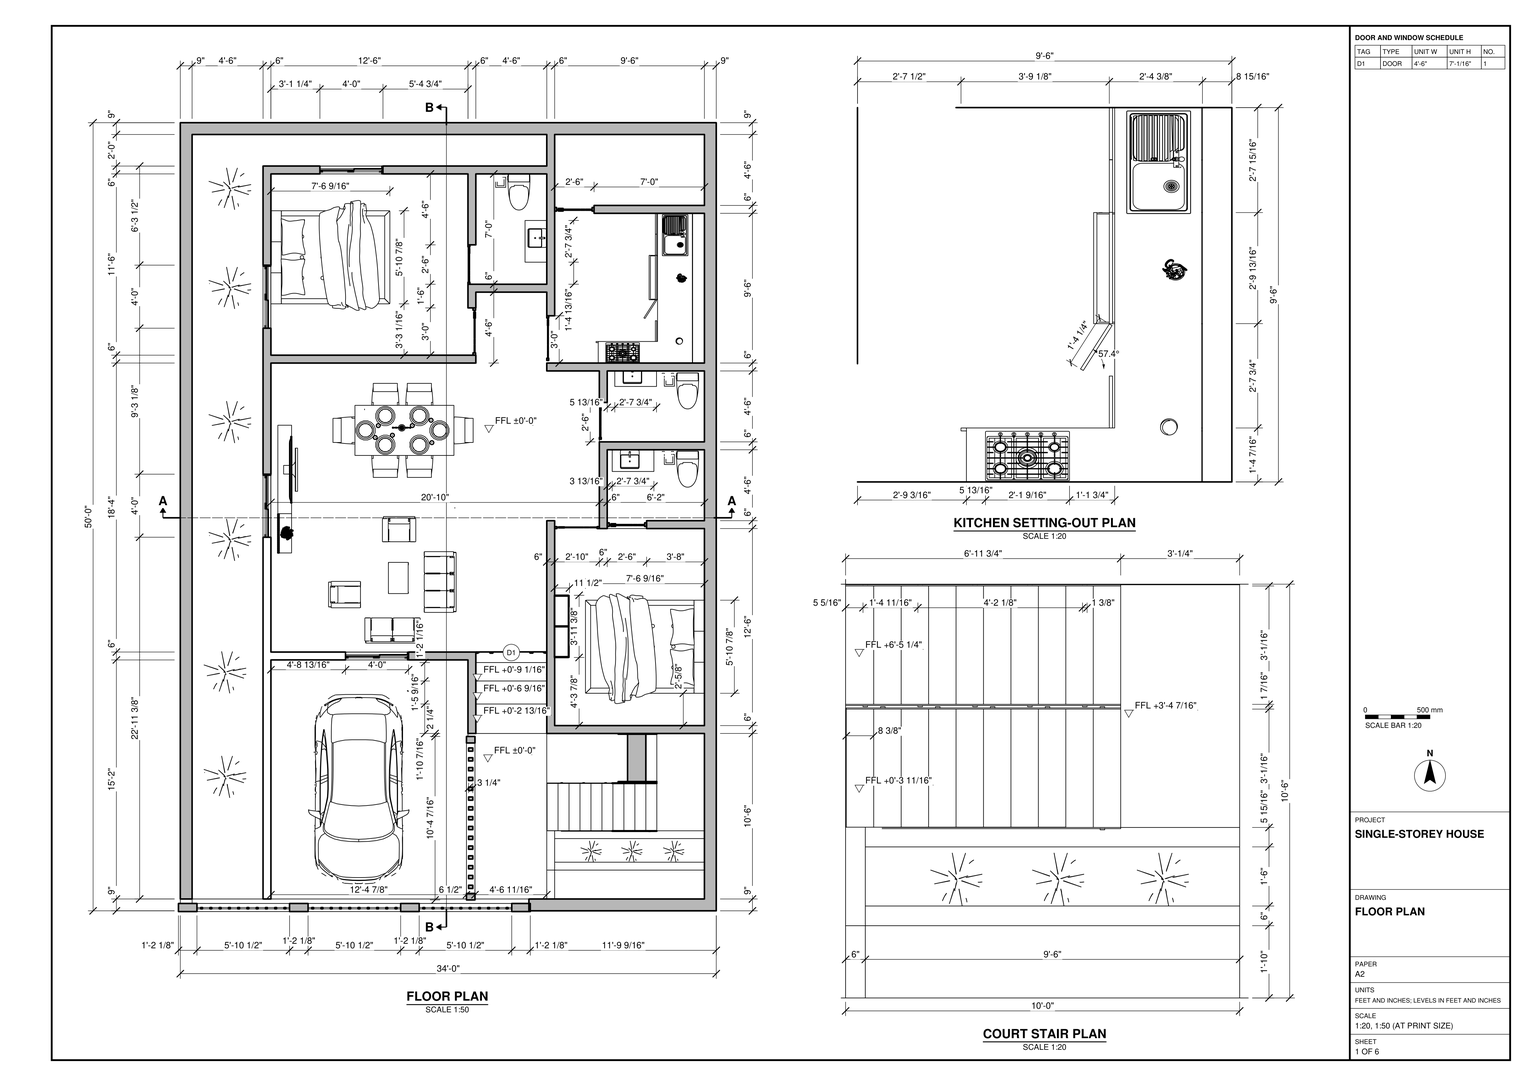
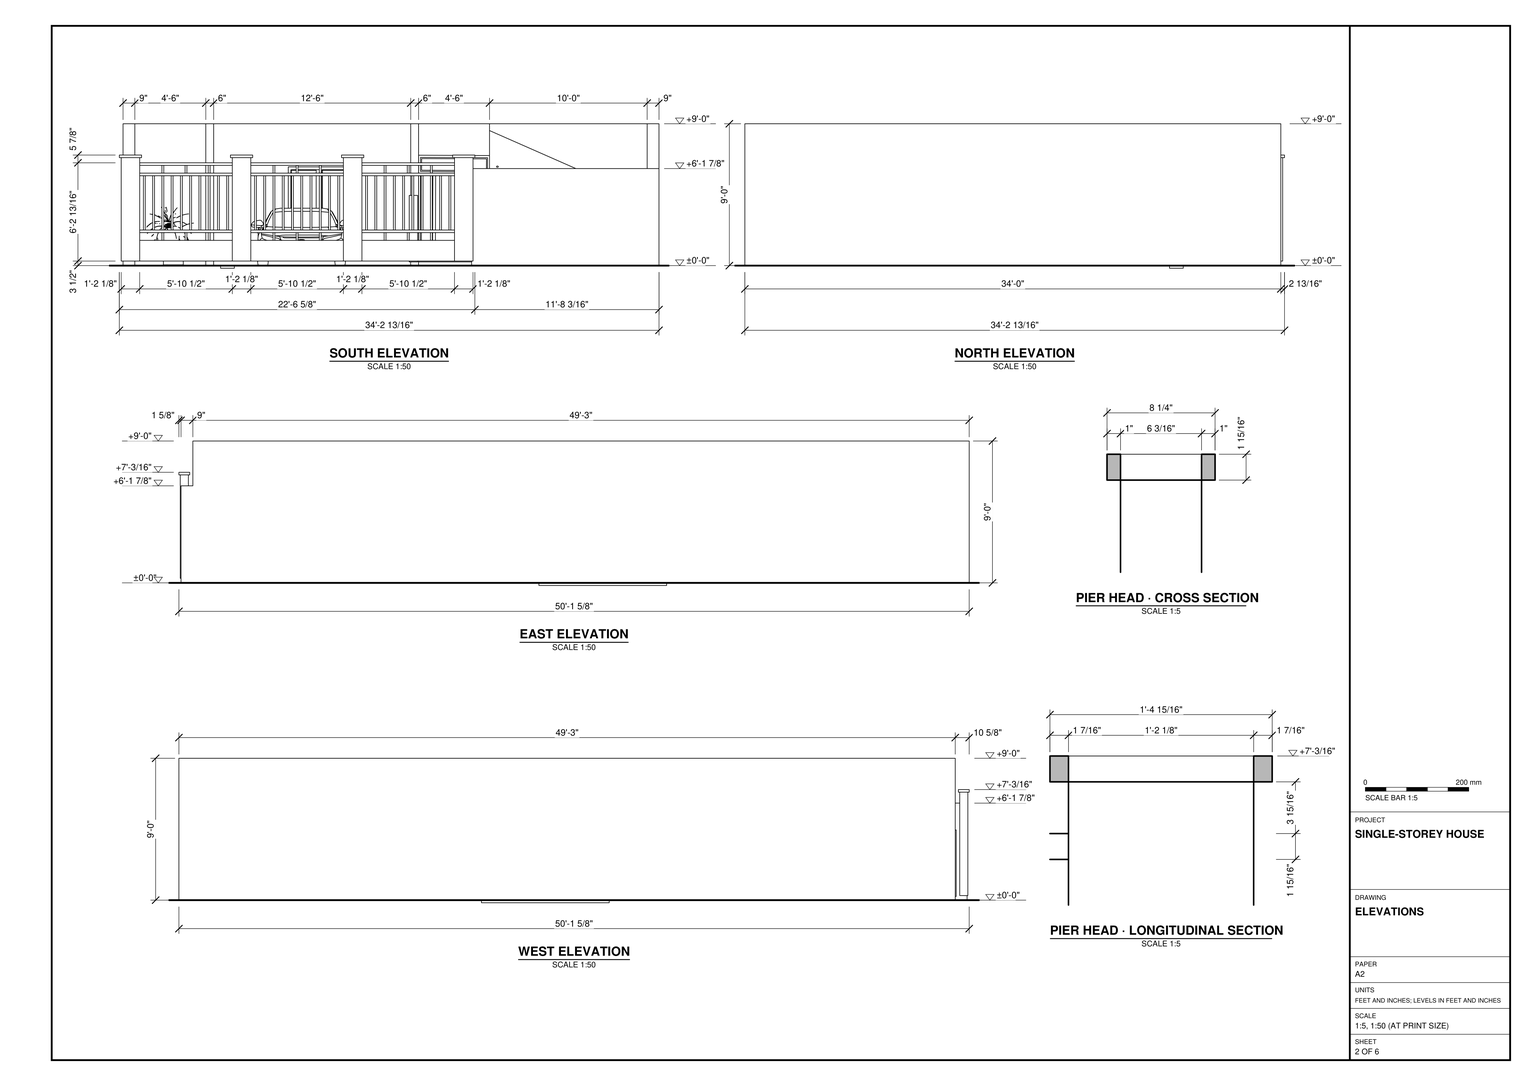
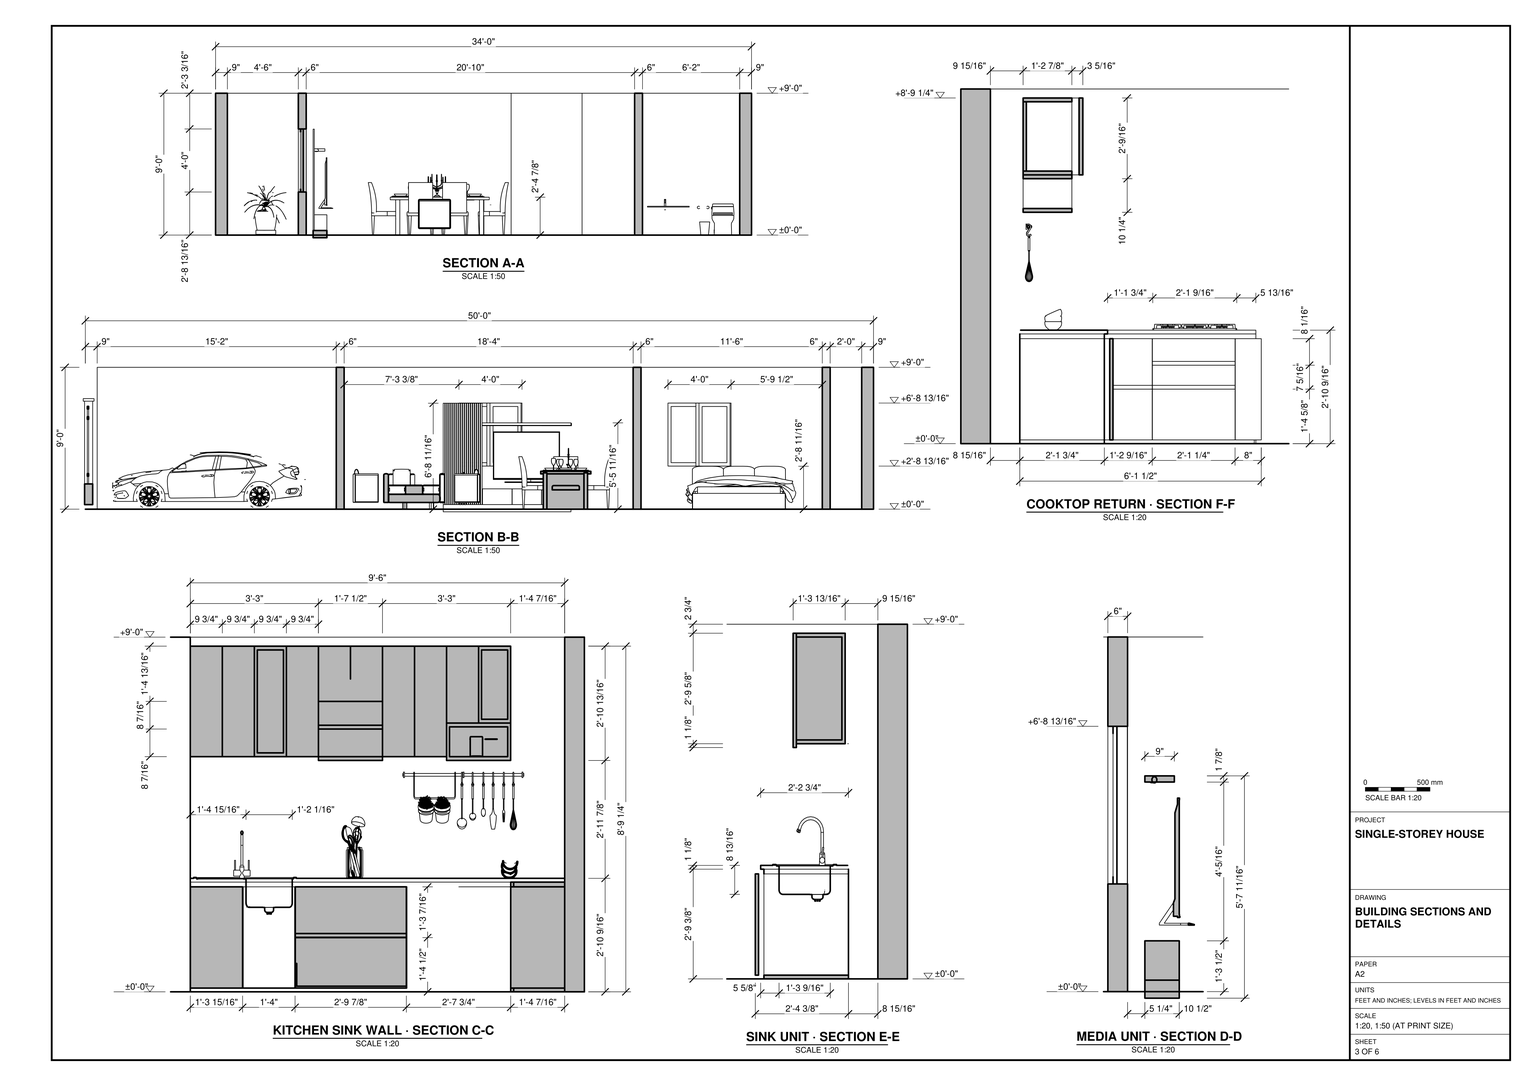
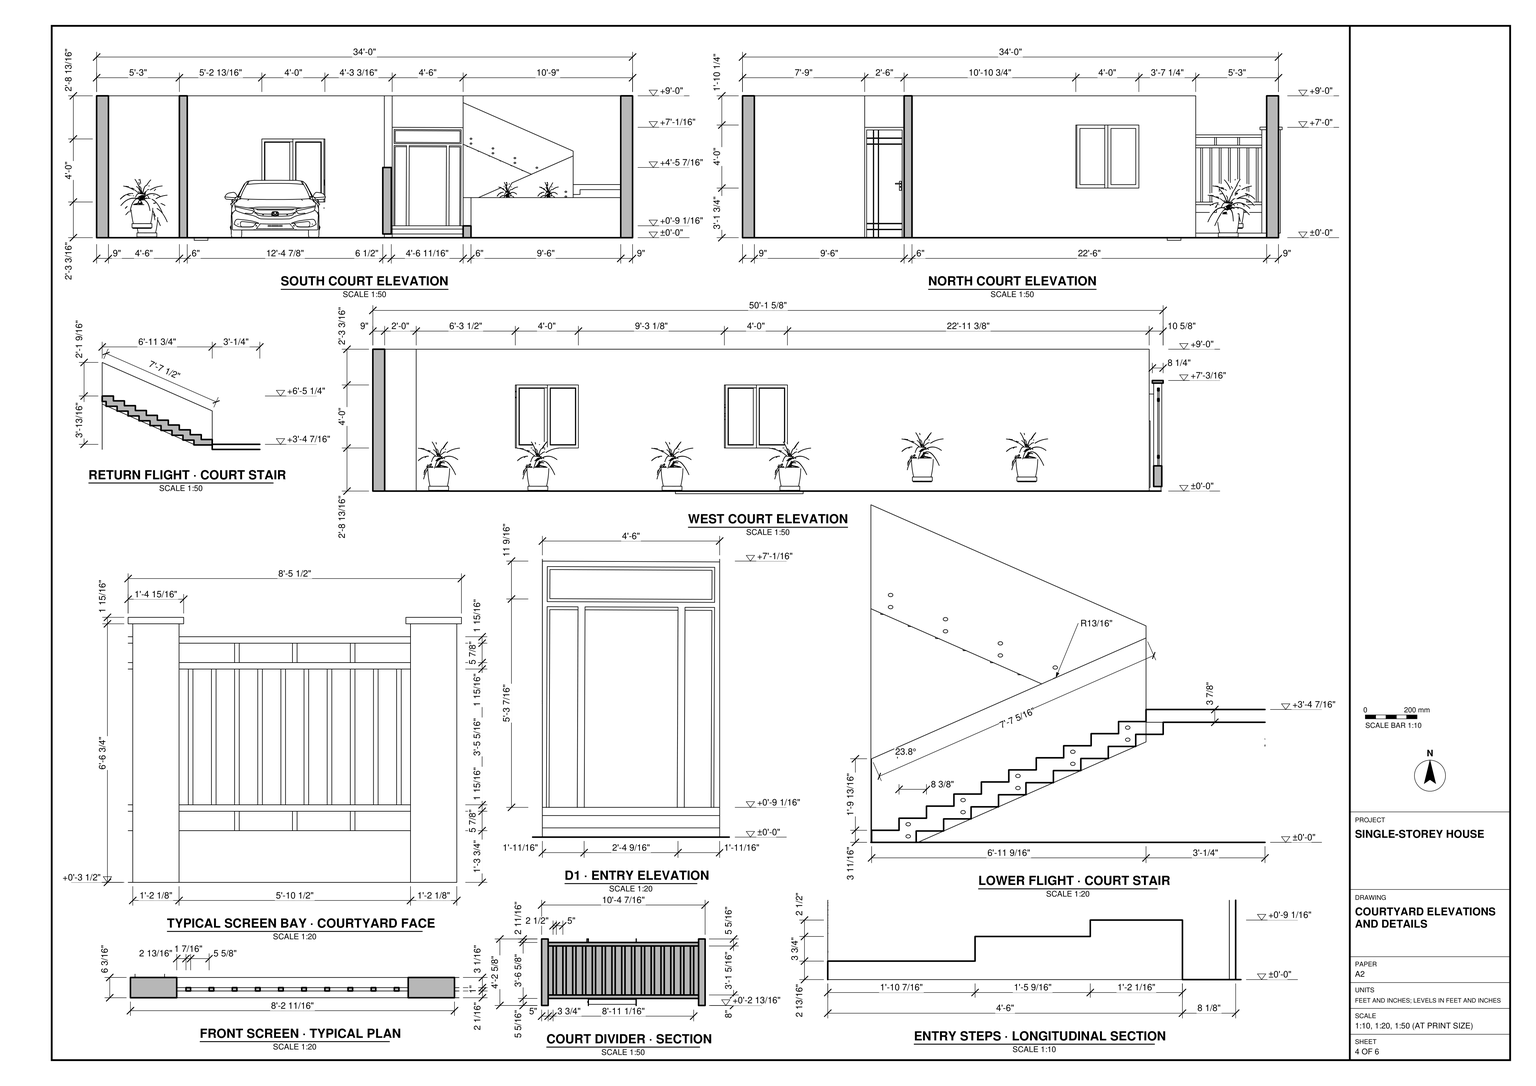
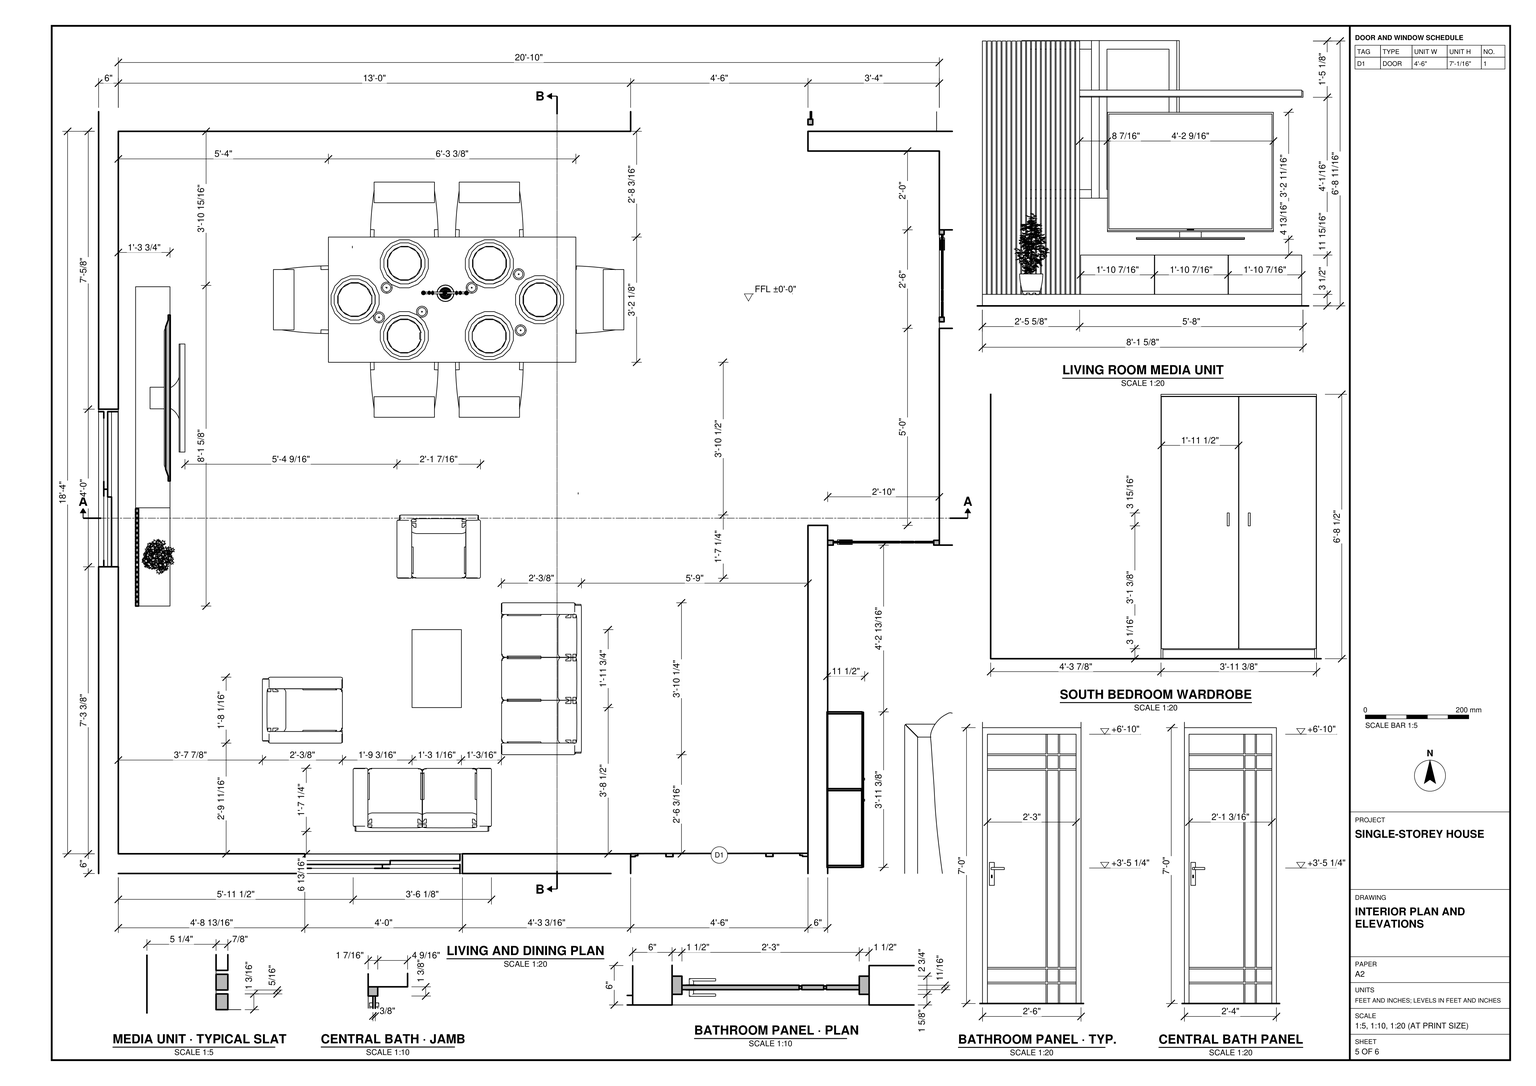
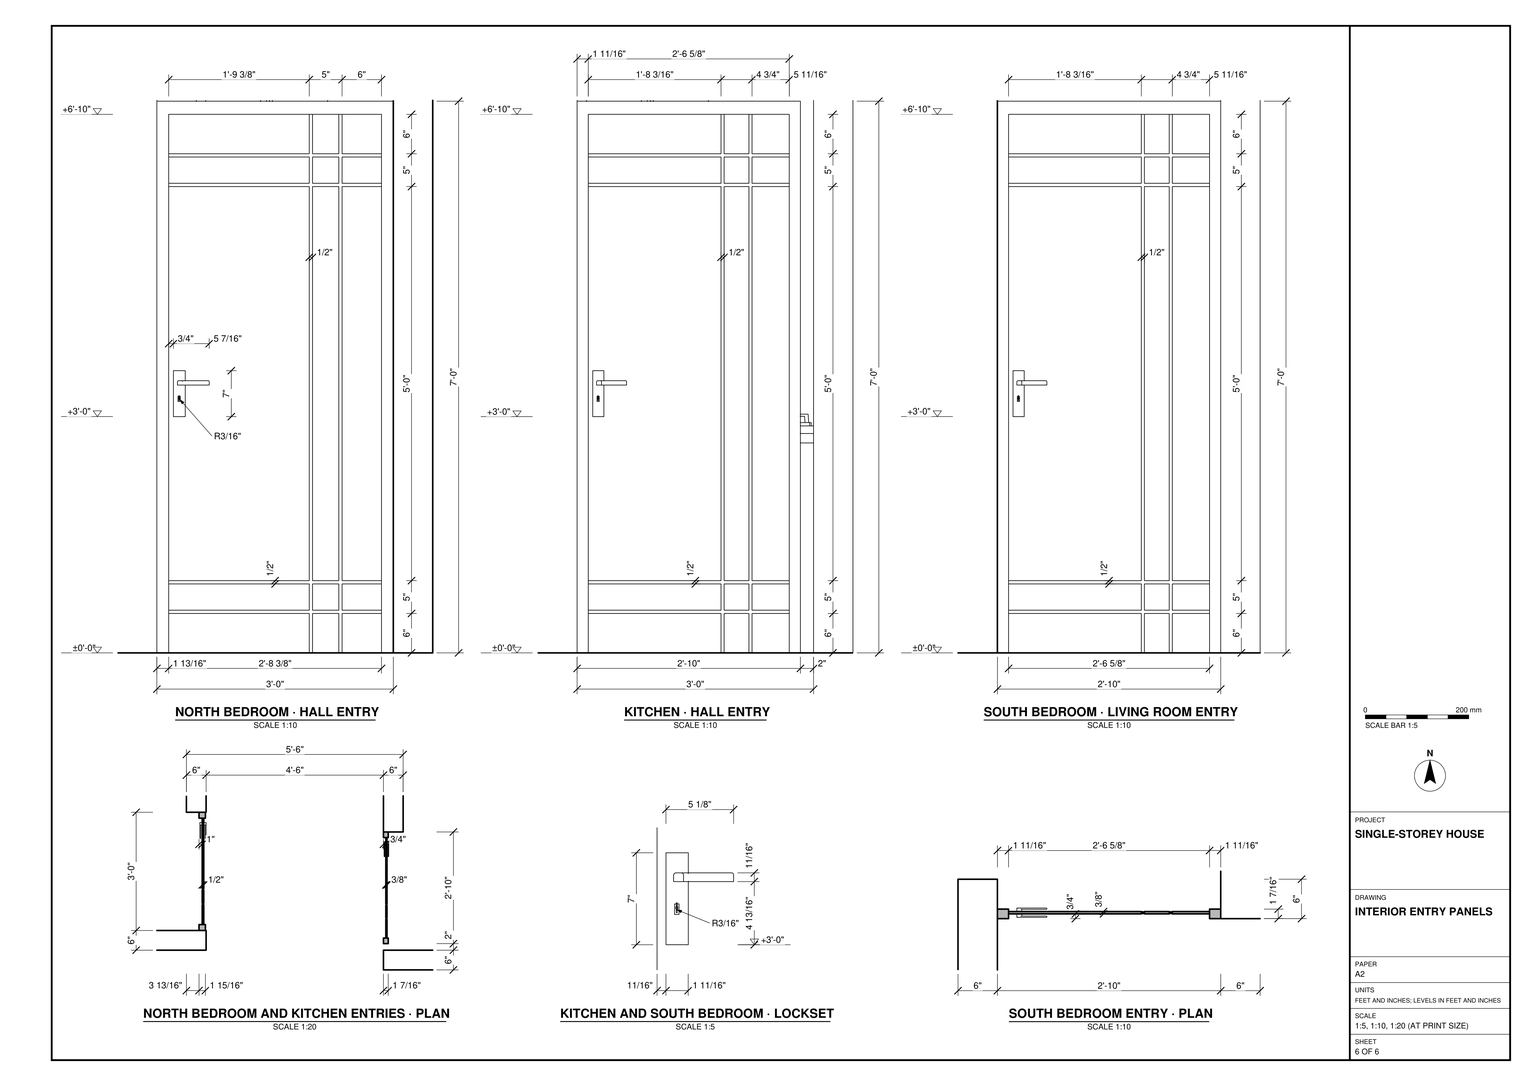
Build the house in SketchUp from task_files/diagram_01.pdf. Work in feet and inches. The complete model, including the front boundary, is 34'-2 13/16" wide, 50'-1 5/8" deep and 9'-2" high. Use ±0'-0" as the ground-floor level; the entrance steps and court stair are local changes in level, not additional storeys.

Set out the floor slabs and walls from the plan, using 9" perimeter walls and 6" partitions where dimensioned. Place the living and dining space between the two bedrooms, with the kitchen to the northeast and the sanitary rooms in their drawn positions. Fit the door and window units into the wall openings. Follow the sections for wall heads, sills and slab edges, and keep the courts open. Include the front parking bay, the planted side passage, the stepped entrance and the separate stair in the southeast court. Match the railed bays, capped piers and solid wall in the south elevation.

Model the kitchen base and wall cabinets, sink counter and cooktop return from the setting-out plan and sections. Include the beds, dining table and chairs, living-room seating, low table, media unit and sanitary fixtures at the sizes and positions shown. Decor and loose items may be any suitable library components.

Keep shell elements and individual furniture and joinery pieces in separate groups or components, and use components for repeated parts. Save one SketchUp model as output_files/single_storey_house_with_a_stair_court.skp.

# SketchUp Ruby script. Lengths in inches.
U = 1.inch
M = Sketchup.active_model
def pt(a) = Geom::Point3d.new(a.map { |v| v * U })
def face(e, loops, mat)
  f = e.add_face(loops[0].map { |a| pt(a) })
  loops[1..].each { |l| e.add_face(l.map { |a| pt(a) }).erase! }
  f.material = f.back_material = mat if mat
  f
end
# faces: each face lists its corners as indices into pts; further lists are holes
def faces(e, pts, list, mat = nil) = list.each { |f| face(e, (f[0].is_a?(Array) ? f : [f]).map { |l| l.map { |i| pts[i] } }, mat) }
# xy, xz, yz: faces in a plane at the given z, y or x. An outline is a flat list of corners, or four numbers for a rectangle; further outlines are holes
def ring(l) = l.size == 4 ? [[l[0], l[1]], [l[2], l[1]], [l[2], l[3]], [l[0], l[3]]] : l.each_slice(2).to_a
def flat(e, list, mat, &to3) = list.each { |f| face(e, (f[0].is_a?(Array) ? f : [f]).map { |l| ring(l).map { |u, v| to3.(u, v) } }, mat) }
def xy(e, z, list, mat = nil) = flat(e, list, mat) { |x, y| [x, y, z] }
def xz(e, y, list, mat = nil) = flat(e, list, mat) { |x, z| [x, y, z] }
def yz(e, x, list, mat = nil) = flat(e, list, mat) { |y, z| [x, y, z] }
def lines(e, pts, list) = list.each { |a, b| e.add_line(pt(pts[a]), pt(pts[b])) }
# prism: a flat outline (further loops are holes) pulled along v
def prism(e, loops, v, mat = nil)
  f = face(e, loops, mat); d = Geom::Vector3d.new(v.map { |x| x * U })
  f.pushpull(f.normal.samedirection?(d) ? d.length : -d.length)
end
def box(e, o, s, mat = nil) = prism(e, [[o, [o[0] + s[0], o[1], o[2]], [o[0] + s[0], o[1] + s[1], o[2]], [o[0], o[1] + s[1], o[2]]]], [0, 0, s[2]], mat)
def at(x, y, z, deg = 0) = Geom::Transformation.translation(pt([x, y, z])) * Geom::Transformation.rotation(ORIGIN, Z_AXIS, deg.degrees)
def axes(o, x, y, z) = Geom::Transformation.new([*x, 0, *y, 0, *z, 0, *pt(o).to_a, 1])
def part(name) = M.definitions.add(name)
# library, detail: a bought-in or finely detailed component or shape, given as its bounding box
def library(name, o, s) = part(name).tap { |d| box(d.entities, o, s) }
def detail(e, o, s) = box(e.add_group.entities, o, s)
def put(e, d, t, mat = nil) = e.add_instance(d, t).tap { |i| i.material = mat if mat }
def group(e, t, mat = nil) = e.add_group.tap { |g| g.transformation = t; g.material = mat if mat }.entities
root = M.entities
M.materials.add("3-Examples-of-Design-of-Three-Wooden-Entrance-Door-with-Side").color = [165, 127, 91]
M.materials.add("[Cladding Siding White]").color = [207, 207, 207]
M.materials.add("[Grass Dark Green]").color = [106, 157, 55]
M.materials.add("[Groundcover Rock Crushed Multi]").color = [143, 133, 129]
M.materials.add("[Marble Carrara Floor Tile]").color = [204, 208, 219]
M.materials.add("[Metal_Aluminum_Anodized]").color = [200, 209, 218]
M.materials.add("[Pavers Flagstone Gray]").color = [162, 162, 162]
M.materials.add("[Pavers with Grass Herringbone]").color = [197, 201, 190]
M.materials.add("[Translucent Glass Blue]").color = [100, 149, 237]
M.materials["[Translucent Glass Blue]"].alpha = 0.5
M.materials.add("[Translucent Glass Gray]").color = [128, 128, 128]
M.materials["[Translucent Glass Gray]"].alpha = 0.5
M.materials.add("[Vegetation Bark Ponderosa]").color = [158, 116, 100]
M.materials.add("[Wood Fence with Lattice]").color = [170, 106, 61]
c1 = part("Agrupar\#1")
detail(c1.entities,[0,0,0],[43.31,13.99,7.25])
c2 = library("Agrupar\#2",[0,0,0],[66.49,2.6,38.28])
c3 = part("Samsung 75")
p = [[0,0,0],[1,0,0],[1,1,0]]
lines(c3.entities,p,[[0,1],[1,2],[2,0]])
put(c3.entities,c1,at(200.625,110.82,-2.44),"[Metal_Aluminum_Anodized]")
put(c3.entities,c2,at(189.03,116.54,0))
c4 = library("Vtufgjkbc",[-37.34,-38.3,0],[76.68,71.13,141.17])
c5 = part("Enscape.LinearLight")
xz(c5.entities,-44.64,[[0,-1,0,0,-0.38,-0.92],[0,-1,0.38,-0.92,0,0],[-0.38,-0.92,0,0,-0.71,-0.71],[0.38,-0.92,0.71,-0.71,0,0],[-0.71,-0.71,0,0,-0.92,-0.38],
  [0.71,-0.71,0.92,-0.38,0,0],[-0.92,-0.38,0,0,-1,0],[0.92,-0.38,1,0,0,0],[-1,0,0,0,-0.92,0.38],[0,0,-0.71,0.71,-0.92,0.38],
  [0,0,-0.38,0.92,-0.71,0.71],[0,0,0,1,-0.38,0.92],[0,0,0.38,0.92,0,1],[0,0,0.71,0.71,0.38,0.92],[0,0,0.92,0.38,0.71,0.71],
  [0,0,1,0,0.92,0.38]])
xz(c5.entities,44.64,[[0,-1,-0.38,-0.92,0,0],[0,-1,0,0,0.38,-0.92],[-0.38,-0.92,-0.71,-0.71,0,0],[0.38,-0.92,0,0,0.71,-0.71],[-0.71,-0.71,-0.92,-0.38,0,0],
  [0.71,-0.71,0,0,0.92,-0.38],[-0.92,-0.38,-1,0,0,0],[0.92,-0.38,0,0,1,0],[-1,0,-0.92,0.38,0,0],[0,0,-0.92,0.38,-0.71,0.71],
  [0,0,-0.71,0.71,-0.38,0.92],[0,0,-0.38,0.92,0,1],[0,0,0,1,0.38,0.92],[0,0,0.38,0.92,0.71,0.71],[0,0,0.71,0.71,0.92,0.38],
  [0,0,0.92,0.38,1,0]])
p = [[-0.38,-44.64,-0.92],[-0.38,44.64,-0.92],[0,44.64,-1],[0,-44.64,-1],[0.38,44.64,-0.92],[0.38,-44.64,-0.92],
  [-0.71,-44.64,-0.71],[-0.71,44.64,-0.71],[0.71,44.64,-0.71],[0.71,-44.64,-0.71],[-0.92,-44.64,-0.38],[-0.92,44.64,-0.38],
  [0.92,44.64,-0.38],[0.92,-44.64,-0.38],[-1,-44.64,0],[-1,44.64,0],[1,44.64,0],[1,-44.64,0],
  [-0.92,-44.64,0.38],[-0.92,44.64,0.38],[0.92,44.64,0.38],[0.92,-44.64,0.38],[-0.71,-44.64,0.71],[-0.71,44.64,0.71],
  [0.71,44.64,0.71],[0.71,-44.64,0.71],[-0.38,-44.64,0.92],[-0.38,44.64,0.92],[0.38,44.64,0.92],[0.38,-44.64,0.92],
  [0,-44.64,1],[0,44.64,1]]
faces(c5.entities,p,[[0,1,2],[0,2,3],[3,2,4],[3,4,5],[6,7,1],[6,1,0],[5,4,8],[5,8,9],
  [10,11,7],[10,7,6],[9,8,12],[9,12,13],[14,15,11],[14,11,10],[13,12,16],[13,16,17],
  [18,19,15],[18,15,14],[17,16,20],[17,20,21],[22,23,19],[22,19,18],[21,20,24],[21,24,25],
  [26,27,23],[26,23,22],[25,24,28],[25,28,29],[30,31,27],[30,27,26],[29,28,31],[29,31,30]])
c6 = part("Group\#8")
box(c6.entities,[0,0,0],[1.57,1.18,81.22])
c7 = part("tv unit")
put(c7.entities,c3,at(-134.98,-45.95,38.54))
put(c7.entities,c4,axes([23.51,76.07,18.38],[0.185,0,0],[0,0.185,0],[0,0,0.185]))
put(c7.entities,c5,axes([87.75,81.2,82.67],[-0.0192,0.99911,-0.03748],[-0.99982,-0.01919,0.00072],[0,0.03749,0.9993]))
g1 = group(c7.entities,at(3.9375,84.65,12.68))
box(g1,[0,-13.78,0],[127.95,13.78,5.79])
g2 = group(c7.entities,at(43.31,84.65,18.46))
prism(g2,[[[0,0,0],[88.58,0,0],[88.58,-13.78,0],[59.21,-13.78,0],[59.21,-12.99,0],[59.06,-12.99,0],[59.06,-13.78,0],[29.69,-13.78,0],[29.69,-12.99,0],[29.53,-12.99,0],[29.53,-13.78,0],[0,-13.78,0]]],[0,0,12.6])
g3 = group(c7.entities,at(3.9375,84.65,18.46))
put(g3,c6,at(0,-1.18,0))
g4 = group(g3,at(1.97,-1.18,0))
box(g4,[0,0,0],[1.57,1.18,81.22])
put(g3,c6,at(3.9375,-1.18,0))
put(g3,c6,at(5.91,-1.18,0))
g5 = group(g3,at(7.875,-1.18,0))
box(g5,[0,0,0],[1.57,1.18,81.22])
put(g3,c6,at(9.84,-1.18,0))
put(g3,c6,at(11.8125,-1.18,0))
put(g3,c6,at(13.78,-1.18,0))
put(g3,c6,at(15.75,-1.18,0))
put(g3,c6,at(17.72,-1.18,0))
put(g3,c6,at(19.69,-1.18,0))
put(g3,c6,at(21.65,-1.18,0))
put(g3,c6,at(23.62,-1.18,0))
g6 = group(g3,at(25.59,-1.18,0))
box(g6,[0,0,0],[1.57,1.18,81.22])
put(g3,c6,at(27.56,-1.18,0))
put(g3,c6,at(29.53,-1.18,0))
put(g3,c6,at(31.5,-1.18,0))
put(g3,c6,at(33.46,-1.18,0))
put(g3,c6,at(35.43,-1.18,0))
put(g3,c6,at(37.4,-1.18,0))
g7 = group(c7.entities,at(42.91,84.65,81.97))
box(g7,[0,-11.8125,0],[88.98,11.8125,1.97])
c8 = library("Шкаф+для+одежды+1",[-0.2,0,0],[17.13,47.36,80.51])
c9 = library("car\#1",[0.01,0.03,0.02],[18.76,39.97,12.32])
c10 = library("Untitled",[0,0,0],[36,4.39,84])
c11 = part("Janela aluminio")
xy(c11.entities,0,[[0,0,47.24,1.57],[23.62,1.57,47.24,2.76],[0,2.76,25.98,3.9375],[0,3.9375,47.24,5.91]])
xy(c11.entities,43.31,[[0,0,47.24,1.57],[23.62,1.57,47.24,2.76],[0,2.76,0,5.91,47.24,5.91,47.24,3.9375,25.98,3.9375,25.98,2.76],[25.98,2.76,47.24,3.9375]])
xz(c11.entities,1.57,[[0,0,23.62,0,23.62,41.34,21.26,41.34,21.26,1.97,1.97,1.97,1.97,41.34,23.62,41.34,23.62,43.31,0,43.31],[[23.62,0,47.24,43.31],[25.7,1.97,45.28,41.34]]])
xz(c11.entities,2.76,[[[0,0,23.62,43.31],[2.36,2.36,21.26,40.94]],[23.62,0,25.98,43.31]])
xz(c11.entities,2.76,[[2.36,2.36,21.26,40.94]],"[Translucent Glass Blue]")
xz(c11.entities,3.9375,[[25.98,0,25.98,2.36,44.88,2.36,44.88,40.94,25.98,40.94,25.98,43.31,47.24,43.31,47.24,0]])
xz(c11.entities,3.9375,[[25.98,2.36,44.88,40.94]],"[Translucent Glass Blue]")
yz(c11.entities,0,[[0,0,1.57,43.31],[2.76,0,5.91,43.31]])
yz(c11.entities,23.62,[[1.57,0,2.76,43.31]])
yz(c11.entities,25.98,[[2.76,0,3.9375,43.31]])
yz(c11.entities,47.24,[[0,0,1.57,43.31],[1.57,0,2.76,43.31],[3.9375,0,5.91,43.31]])
c12 = library("Upholstered double bed",[0,0,0],[90.55,83.75,32.69])
c13 = library("Fence+drawing",[11.65,10.19,0],[100,4,38])
c14 = library("Group\#1437",[0,-3.9375,-72.83],[98.43,11.8125,74.8])
c15 = library("Group\#1441",[0,-3.9375,-72.83],[98.43,11.8125,74.8])
c16 = library("Group\#1442",[0,-3.9375,-72.83],[98.43,11.8125,74.8])
c17 = part("pagar")
p = [[0,0,0],[1,0,0],[1,1,0]]
lines(c17.entities,p,[[0,1],[1,2],[2,0]])
g8 = group(c17.entities,at(0,0,0))
xy(g8,0,[[0,0,19.69,11.8125]])
xy(g8,78.74,[[[-1.97,-1.97,21.65,13.78],[0,0,19.69,11.8125]],[0,0,19.69,11.8125]])
xy(g8,80.71,[[[-1.97,-1.97,21.65,13.78],[0,0,19.69,11.8125]]])
xz(g8,-1.97,[[-1.97,78.74,21.65,80.71]])
xz(g8,0,[[0,0,19.69,78.74],[0,78.74,19.69,80.71]])
xz(g8,11.8125,[[0,0,19.69,78.74],[0,78.74,19.69,80.71]])
xz(g8,13.78,[[-1.97,78.74,21.65,80.71]])
yz(g8,-1.97,[[-1.97,78.74,13.78,80.71]])
yz(g8,0,[[0,0,11.8125,78.74],[0,78.74,11.8125,80.71]])
yz(g8,19.69,[[0,0,11.8125,78.74],[0,78.74,11.8125,80.71]])
yz(g8,21.65,[[-1.97,78.74,13.78,80.71]])
g9 = group(c17.entities,at(118.11,0,0))
xy(g9,0,[[0,0,19.69,11.8125]])
xy(g9,78.74,[[[-1.97,-1.97,21.65,13.78],[0,0,19.69,11.8125]],[0,0,19.69,11.8125]])
xy(g9,80.71,[[[-1.97,-1.97,21.65,13.78],[0,0,19.69,11.8125]]])
xz(g9,-1.97,[[-1.97,78.74,21.65,80.71]])
xz(g9,0,[[0,0,19.69,78.74],[0,78.74,19.69,80.71]])
xz(g9,11.8125,[[0,0,19.69,78.74],[0,78.74,19.69,80.71]])
xz(g9,13.78,[[-1.97,78.74,21.65,80.71]])
yz(g9,-1.97,[[-1.97,78.74,13.78,80.71]])
yz(g9,0,[[0,0,11.8125,78.74],[0,78.74,11.8125,80.71]])
yz(g9,19.69,[[0,0,11.8125,78.74],[0,78.74,11.8125,80.71]])
yz(g9,21.65,[[-1.97,78.74,13.78,80.71]])
g10 = group(c17.entities,at(236.22,0,0))
xy(g10,0,[[0,0,19.69,11.8125]])
xy(g10,78.74,[[[-1.97,-1.97,21.65,13.78],[0,0,19.69,11.8125]],[0,0,19.69,11.8125]])
xy(g10,80.71,[[[-1.97,-1.97,21.65,13.78],[0,0,19.69,11.8125]]])
xz(g10,-1.97,[[-1.97,78.74,21.65,80.71]])
xz(g10,0,[[0,0,19.69,78.74],[0,78.74,19.69,80.71]])
xz(g10,11.8125,[[0,0,19.69,78.74],[0,78.74,19.69,80.71]])
xz(g10,13.78,[[-1.97,78.74,21.65,80.71]])
yz(g10,-1.97,[[-1.97,78.74,13.78,80.71]])
yz(g10,0,[[0,0,11.8125,78.74],[0,78.74,11.8125,80.71]])
yz(g10,19.69,[[0,0,11.8125,78.74],[0,78.74,11.8125,80.71]])
yz(g10,21.65,[[-1.97,78.74,13.78,80.71]])
g11 = group(c17.entities,at(354.33,0,0))
xy(g11,0,[[0,0,19.69,11.8125]])
xy(g11,78.74,[[[-1.97,-1.97,21.65,13.78],[0,0,19.69,11.8125]],[0,0,19.69,11.8125]])
xy(g11,80.71,[[[-1.97,-1.97,21.65,13.78],[0,0,19.69,11.8125]]])
xz(g11,-1.97,[[-1.97,78.74,21.65,80.71]])
xz(g11,0,[[0,0,19.69,78.74],[0,78.74,19.69,80.71]])
xz(g11,11.8125,[[0,0,19.69,78.74],[0,78.74,19.69,80.71]])
xz(g11,13.78,[[-1.97,78.74,21.65,80.71]])
yz(g11,-1.97,[[-1.97,78.74,13.78,80.71]])
yz(g11,0,[[0,0,11.8125,78.74],[0,78.74,11.8125,80.71]])
yz(g11,19.69,[[0,0,11.8125,78.74],[0,78.74,11.8125,80.71]])
yz(g11,21.65,[[-1.97,78.74,13.78,80.71]])
put(c17.entities,c14,at(19.69,3.9375,72.83))
put(c17.entities,c15,at(137.8,3.9375,72.83))
put(c17.entities,c16,at(255.91,3.9375,72.83))
c18 = library("4",[-16.3,-15.81,0],[32.6,31.62,37.8])
c19 = library("Dining Table",[54.55,57.53,0],[71.62,106.71,46.43])
c20 = library("Kitchen+with+cabinets",[0,0,0],[74.29,127.68,91.13])
c21 = part("Main+Door+1")
xy(c21.entities,0,[[0,0,-0.01,2.95,2.1875,2.96,2.2,0.99,1.29,0.99,1.3,0.01],[11.72,0.05,11.71,3,14.07,3.01,14.08,0.06],[45.45,0.19,45.4375,3.15,47.8,3.16,47.8125,0.2],[57.78,0.25,57.78,1.23,56.875,1.23,56.87,3.19,59.78,3.21,59.79,0.25]])
p = [[-0.01,2.95,84.06],[-0.01,2.95,0],[0,0,0],[0,0,84.06],[1.3,0.01,0],[1.59,0.01,70.18],
  [12.02,0.05,70.14],[11.72,0.05,0],[14.08,0.06,0],[14.38,0.0625,70.13],[45.75,0.19,70],[45.74,0.19,68.3],
  [45.45,0.19,0],[47.8125,0.2,0],[48.1,0.2,68.29],[48.11,0.2,69.99],[58.08,0.25,69.94],[57.78,0.25,0],
  [59.79,0.25,0],[59.79,0.25,83.8],[58.13,0.25,82.16],[58.09,0.25,71.48],[1.6,0.01,71.72],[1.65,0.01,82.4],
  [1.29,0.99,0],[1.59,0.99,70.18],[12,3,69.23],[11.71,3,0],[12.01,1.04,70.14],[12.01,1.04,69.23],
  [14.07,3.01,0],[14.36,3.01,69.22],[14.37,1.05,69.22],[14.375,1.05,70.13],[45.73,3.15,69.09],[45.4375,3.15,0],
  [45.74,1.18,69.09],[47.8,3.16,0],[48.09,3.16,69.08],[48.1,1.1875,69.08],[58.08,1.23,69.94],[57.78,1.23,0],
  [59.78,3.21,0],[59.78,3.21,83.8],[2.2,0.99,0],[2.49,0.99,69.27],[2.1875,2.96,0],[2.48,2.96,69.27],
  [57.17,1.23,69.04],[56.875,1.23,0],[48.11,1.1875,69.99],[57.16,3.2,69.04],[56.87,3.19,0],[2.5,2.96,72.62],
  [2.54,2.96,81.49],[57.21,3.2,81.25],[57.17,3.2,72.39],[45.74,1.18,70],[58.08,1.23,71.48],[1.6,0.99,71.72],
  [58.13,1.23,82.16],[1.64,0.99,82.4],[2.51,0.99,72.62],[2.54,1,81.49],[57.22,1.23,81.25],[57.18,1.23,72.39]]
faces(c21.entities,p,[[0,1,2,3],[[3,2,4,5,6,7,8,9,10,11,12,13,14,15,16,17,18,19],[20,21,22,23]],[5,4,24,25],[26,27,7,6,28,29],[9,8,30,31,32,33],[34,35,12,11,36],[14,13,37,38,39],[40,41,17,16],
  [19,18,42,43],[25,24,44,45,29,28],[45,44,46,47],[48,49,41,40,50,39],[51,52,49,48],[[35,37,38,51,52,42,43,0,1,46,47,26,27,30,31,34],[53,54,55,56]],[47,46,27,26],[38,37,52,51],
  [57,36,11,10],[39,50,15,14],[48,39,38,51],[31,34,36,32],[32,36,57,33],[47,26,29,45],[16,15,50,40],[57,10,9,33],
  [28,6,5,25],[21,58,59,22],[20,60,58,21],[[58,60,61,59],[62,63,64,65]],[22,59,61,23],[56,53,62,65],[55,56,65,64],[54,53,56,55],
  [53,54,63,62],[54,55,64,63],[23,61,60,20],[43,0,3,19]],"3-Examples-of-Design-of-Three-Wooden-Entrance-Door-with-Side")
g12 = group(c21.entities,at(14.07,3.01,0))
p = [[0.29,0,69.22],[0,0,0],[31.37,0.13,0],[31.66,0.13,69.09]]
faces(g12,p,[[0,1,2,3]],"3-Examples-of-Design-of-Three-Wooden-Entrance-Door-with-Side")
c22 = library("Group\#35",[0,0,0],[160.51,127.83,29.04])
c23 = library("Group\#1451",[0,0,0],[98,1,65.82])
c24 = library("Group\#1448",[0,0,0],[98,1,65.82])
c25 = library("Group\#1452",[0,0,0],[98,51.75,65.8])
c26 = part("Group\#1443")
prism(c26.entities,[[[0,0.5,49.09],[120,0.5,120],[120,0.5,58.98],[20.19,0.5,0],[0,0.5,0]]],[0,-0.5,0],"[Translucent Glass Gray]")
c27 = library("Group\#1449",[0,-102.5,0],[174.3,102.5,148.91])
c28 = library("Group\#1490",[0.07,0,0],[27.9,27.42,23.87])
c29 = library("Group\#1495",[0,0,0],[56.7,23.65,11.32])
xy(root,0,[[2.81,1.61,11.81,10.61],[[268.2,1.61,268.2,10.61,281.81,10.61,281.81,62.61,401.81,62.61,401.81,56.61,287.81,56.61,287.81,38.61,401.81,38.61,401.81,136.61,281.81,136.61,281.81,298.61,287.81,298.61,287.81,142.61,401.81,142.61,401.81,292.61,357.81,292.61,357.81,298.61,401.81,298.61,401.81,352.61,327.81,352.61,327.81,292.61,321.81,292.61,321.81,358.61,401.81,358.61,401.81,412.61,327.81,412.61,327.81,388.61,321.81,388.61,321.81,412.61,281.81,412.61,281.81,418.61,401.81,418.61,401.81,532.61,317.81,532.61,317.81,538.61,401.81,538.61,401.81,592.61,287.81,592.61,287.81,454.61,281.81,454.61,281.81,472.61,227.81,472.61,227.81,460.61,221.81,460.61,221.81,478.61,281.81,478.61,281.81,562.61,227.81,562.61,227.81,508.61,221.81,508.61,221.81,562.61,71.81,562.61,71.81,424.61,227.81,424.61,227.81,418.61,71.81,418.61,71.81,198.61,227.81,198.61,227.81,136.61,221.81,136.61,221.81,192.61,71.81,192.61,71.81,10.61,65.81,10.61,65.81,568.61,281.81,568.61,281.81,592.61,11.81,592.61,11.81,10.61,2.81,10.61,2.81,601.61,410.81,601.61,410.81,1.61],[287.81,10.61,401.81,32.61]],[11.81,1.61,268.2,10.61],[71.81,10.61,221.81,192.61],[221.81,10.61,281.81,136.61],
  [287.81,142.61,401.81,142.61,401.81,292.61,321.81,292.61,321.81,412.61,281.81,412.61,281.81,418.61,401.81,418.61,401.81,532.61,317.81,532.61,317.81,538.61,401.81,538.61,401.81,592.61,287.81,592.61,287.81,454.61,281.81,454.61,281.81,472.61,227.81,472.61,227.81,460.61,221.81,460.61,221.81,562.61,71.81,562.61,71.81,424.61,227.81,424.61,227.81,418.61,71.81,418.61,71.81,198.61,227.81,198.61,227.81,190.61,281.81,190.61,281.81,298.61,287.81,298.61],[327.81,292.61,357.81,292.61,357.81,298.61,401.81,298.61,401.81,352.61,327.81,352.61],[321.81,358.61,401.81,358.61,401.81,412.61,327.81,412.61,327.81,388.61,321.81,388.61],[221.81,478.61,281.81,478.61,281.81,562.61,227.81,562.61,227.81,508.61,221.81,508.61]])
xy(root,0,[[287.81,10.61,401.81,32.61]],"[Cladding Siding White]")
xy(root,0,[[11.81,10.61,65.81,10.61,65.81,568.61,281.81,568.61,281.81,592.61,11.81,592.61],[287.81,38.61,401.81,56.61]],"[Grass Dark Green]")
xy(root,0,[[281.81,62.61,401.81,136.61]],"[Pavers Flagstone Gray]")
xy(root,2.8125,[[227.81,136.61,281.81,159.04]])
xy(root,6.5625,[[227.81,159.04,281.81,176.58]])
xy(root,9,[[281.81,10.61,287.81,32.61]])
xy(root,9.0625,[[227.81,176.58,281.81,190.61]])
xy(root,27.17,[[128.59,192.61,176.59,198.61]])
xy(root,30.5,[[281.81,32.61,287.81,62.61],[287.81,32.61,401.81,38.61],[287.81,56.61,401.81,62.61]])
xy(root,32.8,[[65.81,286,71.81,334],[65.81,445.14,71.81,493.14]])
xy(root,37.77,[[109.09,562.61,157.09,568.61]])
xy(root,73.875,[[268.2,1.61,410.81,10.61]])
xy(root,75.17,[[128.59,192.61,176.59,198.61]])
xy(root,80.8,[[65.81,286,71.81,334],[65.81,445.14,71.81,493.14]])
xy(root,85.77,[[109.09,562.61,157.09,568.61]])
xy(root,108,[[2.81,10.61,11.81,10.61,11.81,592.61,281.81,592.61,281.81,568.61,65.81,568.61,65.81,10.61,71.81,10.61,71.81,192.61,221.81,192.61,221.81,136.61,227.81,136.61,227.81,198.61,71.81,198.61,71.81,418.61,227.81,418.61,227.81,424.61,71.81,424.61,71.81,562.61,221.81,562.61,221.81,508.61,227.81,508.61,227.81,562.61,281.81,562.61,281.81,478.61,221.81,478.61,221.81,460.61,227.81,460.61,227.81,472.61,281.81,472.61,281.81,454.61,287.81,454.61,287.81,592.61,401.81,592.61,401.81,538.61,317.81,538.61,317.81,532.61,401.81,532.61,401.81,418.61,281.81,418.61,281.81,412.61,321.81,412.61,321.81,388.61,327.81,388.61,327.81,412.61,401.81,412.61,401.81,358.61,321.81,358.61,321.81,292.61,327.81,292.61,327.81,352.61,401.81,352.61,401.81,298.61,357.81,298.61,357.81,292.61,401.81,292.61,401.81,142.61,287.81,142.61,287.81,298.61,281.81,298.61,281.81,136.61,410.81,136.61,410.81,601.61,2.81,601.61],[401.81,10.61,410.81,136.61]])
xz(root,1.61,[[268.2,0,410.81,73.875]])
xz(root,10.61,[[2.81,0,11.81,108],[65.81,0,71.81,108],[268.2,0,268.2,73.875,401.81,73.875,401.81,0,287.81,0,287.81,9,281.81,9,281.81,0],[401.81,73.875,410.81,108]])
xz(root,32.61,[[287.81,0,401.81,30.5],[281.81,9,287.81,30.5]])
xz(root,38.61,[[287.81,0,401.81,30.5]])
xz(root,56.61,[[287.81,0,401.81,30.5]])
xz(root,62.61,[[281.81,0,401.81,30.5]])
xz(root,136.61,[[221.81,0,227.81,108],[227.81,0,281.81,2.8125]])
xz(root,136.61,[[281.81,0,401.81,108]],"[Pavers with Grass Herringbone]")
xz(root,142.61,[[287.81,0,401.81,108]])
xz(root,159.04,[[227.81,2.8125,281.81,6.5625]])
xz(root,176.58,[[227.81,6.5625,281.81,9.0625]])
xz(root,190.61,[[227.81,0,281.81,9.0625]])
xz(root,192.61,[[[71.81,0,221.81,108],[128.59,27.17,176.59,75.17]]],"[Groundcover Rock Crushed Multi]")
xz(root,198.61,[[[71.81,0,227.81,108],[128.59,27.17,176.59,75.17]]])
xz(root,286,[[65.81,32.8,71.81,80.8]])
xz(root,292.61,[[321.81,0,327.81,108],[357.81,0,401.81,108]])
xz(root,298.61,[[281.81,0,287.81,108]])
xz(root,298.61,[[357.81,0,401.81,108]],"[Marble Carrara Floor Tile]")
xz(root,334,[[65.81,32.8,71.81,80.8]])
xz(root,352.61,[[327.81,0,401.81,108]],"[Marble Carrara Floor Tile]")
xz(root,358.61,[[321.81,0,401.81,108]],"[Marble Carrara Floor Tile]")
xz(root,388.61,[[321.81,0,327.81,108]])
xz(root,412.61,[[327.81,0,401.81,108]],"[Marble Carrara Floor Tile]")
xz(root,412.61,[[281.81,0,321.81,108]],"[Vegetation Bark Ponderosa]")
xz(root,418.61,[[281.81,0,401.81,108]])
xz(root,418.61,[[71.81,0,227.81,108]],"[Wood Fence with Lattice]")
xz(root,424.61,[[71.81,0,227.81,108]])
xz(root,445.14,[[65.81,32.8,71.81,80.8]])
xz(root,454.61,[[281.81,0,287.81,108]])
xz(root,460.61,[[221.81,0,227.81,108]])
xz(root,472.61,[[227.81,0,281.81,108]],"[Vegetation Bark Ponderosa]")
xz(root,478.61,[[221.81,0,281.81,108]])
xz(root,493.14,[[65.81,32.8,71.81,80.8]])
xz(root,508.61,[[221.81,0,227.81,108]])
xz(root,532.61,[[317.81,0,401.81,108]])
xz(root,538.61,[[317.81,0,401.81,108]])
xz(root,562.61,[[[71.81,0,221.81,108],[109.09,37.77,157.09,85.77]]])
xz(root,562.61,[[227.81,0,281.81,108]],"[Marble Carrara Floor Tile]")
xz(root,568.61,[[[65.81,0,281.81,108],[109.09,37.77,157.09,85.77]]])
xz(root,592.61,[[11.81,0,281.81,108],[287.81,0,401.81,108]])
xz(root,601.61,[[2.81,0,410.81,108]])
yz(root,2.81,[[10.61,0,601.61,108]])
yz(root,11.81,[[10.61,0,592.61,108]])
yz(root,65.81,[[[10.61,0,568.61,108],[286,32.8,334,80.8],[445.14,32.8,493.14,80.8]]])
yz(root,71.81,[[10.61,0,192.61,108],[[198.61,0,418.61,108],[286,32.8,334,80.8]],[[424.61,0,562.61,108],[445.14,32.8,493.14,80.8]]])
yz(root,109.09,[[562.61,37.77,568.61,85.77]])
yz(root,128.59,[[192.61,27.17,198.61,75.17]])
yz(root,157.09,[[562.61,37.77,568.61,85.77]])
yz(root,176.59,[[192.61,27.17,198.61,75.17]])
yz(root,221.81,[[136.61,0,192.61,108],[460.61,0,478.61,108],[508.61,0,562.61,108]])
yz(root,227.81,[[136.61,0,190.61,0,190.61,9.0625,176.58,9.0625,176.58,6.5625,159.04,6.5625,159.04,2.8125,136.61,2.8125],[190.61,0,198.61,0,198.61,108,136.61,108,136.61,2.8125,159.04,2.8125,159.04,6.5625,176.58,6.5625,176.58,9.0625,190.61,9.0625],[418.61,0,424.61,108],[460.61,0,472.61,108],[508.61,0,562.61,108]])
yz(root,268.2,[[1.61,0,10.61,73.875]])
yz(root,281.81,[[10.61,0,10.61,9,32.61,9,32.61,30.5,62.61,30.5,62.61,0],[136.61,0,136.61,2.8125,159.04,2.8125,159.04,6.5625,176.58,6.5625,176.58,9.0625,190.61,9.0625,190.61,0],[190.61,0,190.61,9.0625,176.58,9.0625,176.58,6.5625,159.04,6.5625,159.04,2.8125,136.61,2.8125,136.61,108,298.61,108,298.61,0],[412.61,0,418.61,108],[454.61,0,472.61,108],
  [568.61,0,592.61,108]])
yz(root,281.81,[[478.61,0,562.61,108]],"[Marble Carrara Floor Tile]")
yz(root,287.81,[[10.61,0,17.61,9],[17.61,0,20.61,9],[20.61,0,32.61,9],[38.61,0,56.61,30.5],[142.61,0,298.61,108],
  [454.61,0,592.61,108]])
yz(root,317.81,[[532.61,0,538.61,108]])
yz(root,321.81,[[292.61,0,358.61,108],[388.61,0,412.61,108]])
yz(root,327.81,[[292.61,0,352.61,108],[388.61,0,412.61,108]])
yz(root,357.81,[[292.61,0,298.61,108]])
yz(root,401.81,[[56.61,0,62.61,30.5],[142.61,0,292.61,108],[418.61,0,532.61,108],[538.61,0,592.61,108]])
yz(root,401.81,[[298.61,0,352.61,108],[358.61,0,412.61,108]],"[Marble Carrara Floor Tile]")
yz(root,401.81,[[10.61,0,10.61,108,136.61,108,136.61,0,62.61,0,62.61,30.5,56.61,30.5,56.61,0,38.61,0,38.61,30.5,32.61,30.5,32.61,0]],"[Pavers with Grass Herringbone]")
yz(root,410.81,[[1.61,0,601.61,0,601.61,108,10.61,108,10.61,73.875,1.61,73.875]])
p = [[212.42,337.74,22.99],[212.42,337.74,23.04],[211.83,338.21,22.99],[211.83,338.21,23.04],[211.83,337.74,22.99],[211.83,337.74,23.04],
  [212.42,338.21,23.04],[212.42,338.21,22.99],[211.83,308.59,22.99],[211.83,308.12,22.99],[211.83,308.59,23.04],[211.83,308.12,23.04],
  [212.42,308.59,23.04],[212.42,308.59,22.99]]
lines(root,p,[[0,1],[2,3],[4,5],[6,7],[8,9],[8,10],[9,11],[12,13]])
put(root,c7,axes([141.4,271.06,-14.03],[0,0.76,0],[-0.76,0,0],[0,0,0.95]))
put(root,c8,axes([287.74,194.47,0],[0.67,0,0],[0,1,0],[0,0,1]))
put(root,c9,axes([100.25,21.82,-0.06],[4.095,0,0],[0,3.612,0],[0,0,3.54551]))
put(root,c10,axes([327.81,293.93,0],[0.83333,0,0],[0,0.7,0],[0,0,1]))
put(root,c10,axes([287.81,294.22,0],[0.94444,0,0],[0,-0.36747,0],[0,0,1]))
put(root,c10,axes([283.42,454.61,0],[0,-0.94444,0],[-0.36747,0,0],[0,0,1]))
put(root,c10,axes([227.81,460.61,0],[0,-1,0],[-0.49229,0,0],[0,0,1]))
put(root,c10,axes([223.42,508.61,0],[0,-0.83333,0],[-0.36747,0,0],[0,0,1]))
put(root,c10,axes([287.81,533.99,0],[0.83333,0,0],[0,0.7,0],[0,0,1]))
put(root,c11,axes([128.59,192.61,27.17],[1,0,0],[0,1,0],[0,0,1.10836]))
put(root,c11,axes([109.09,562.61,37.77],[1,0,0],[0,1,0],[0,0,1.10836]))
put(root,c11,axes([65.81,492.38,32.8],[0,-1,0],[1,0,0],[0,0,1.10836]))
put(root,c11,axes([65.81,333.25,32.8],[0,-1,0],[1,0,0],[0,0,1.10836]))
put(root,c12,at(71.81,458.67,0))
put(root,c12,at(401.81,243.12,0,-180))
put(root,c13,axes([204.16,-4.61,2.8125],[0,1.2446,0],[1.6191,0,0],[0,0,1.3321]))
put(root,c17,axes([1.41,1.03,3.47],[0.7161,0,0],[0,0.52229,0],[0,0,1]))
put(root,c18,at(37.11,103.59,7.03))
put(root,c18,at(37.11,183.15,7.03))
put(root,c18,at(40.86,284.01,0))
put(root,c18,at(40.86,373.7,0))
put(root,c18,at(40.86,475.82,0))
put(root,c18,at(40.86,551.32,0))
put(root,c18,axes([315.68,46.67,15.95],[0.49,0,0],[0,0.51019,0],[0,0,0.7]))
put(root,c18,axes([346.68,46.67,15.95],[0.49,0,0],[0,0.51019,0],[0,0,0.7]))
put(root,c18,axes([378.55,46.67,4.04],[0.49,0,0],[0,0.51019,0],[0,0,0.7]))
put(root,c10,axes([323.42,388.61,0],[0,-0.77778,0],[-0.36747,0,0],[0,0,1]))
put(root,c19,at(61.5,457.71,0,-90))
put(root,c20,axes([319.33,418.61,0],[0.99,0,0],[0,0.89284,0],[0,0,1.155]))
put(root,c21,axes([227.84,197.74,0],[0.90258,0,0],[0,0.3168,0],[0,0,1]))
put(root,c22,axes([115.67,301.78,0],[0,-0.6004,0],[0.76,0,0],[0,0,1.0488]))
put(root,c23,axes([292.46,61.8,1.32],[0.69635,0,0],[0,0.72103,0],[0,0,0.51875]),"[Pavers Flagstone Gray]")
put(root,c24,axes([292.46,98.58,1.32],[0.69635,0,0],[0,0.72103,0],[0,0,0.51875]),"[Pavers Flagstone Gray]")
put(root,c25,axes([287.11,99.3,41.71],[0.69635,0,0],[0,0.72103,0],[0,0,0.51875]),"[Pavers Flagstone Gray]")
g13 = group(root,at(282.02,62.16,0),"[Pavers Flagstone Gray]")
g14 = group(g13,at(0.7,73.91,40.25))
prism(g14,[[[82.87,0,25.68],[-0.91,0,62.55],[-0.91,0,30.9],[69.29,0,0],[82.87,0,0]]],[0,0.36,0],"[Translucent Glass Gray]")
put(g13,c26,axes([0,36.41,0],[0.69635,0,0],[0,0.72103,0],[0,0,0.51875]))
put(g13,c26,axes([0,0,0],[0.69635,0,0],[0,0.72103,0],[0,0,0.51875]))
g15 = group(g13,at(0.7,37.49,40.25))
prism(g15,[[[82.87,0,25.68],[-0.91,0,62.55],[-0.91,0,30.9],[69.29,0,0],[82.87,0,0]]],[0,0.36,0],"[Translucent Glass Gray]")
put(root,c27,axes([403.18,62.52,0],[-0.69635,0,0],[0,-0.72103,0],[0,0,0.51875]),"[Pavers Flagstone Gray]")
put(root,c28,at(369.44,383.71,0))
put(root,c28,at(369.44,324.15,0))
put(root,c28,at(241.01,535.13,0))
put(root,c29,axes([365.34,417.36,26.78],[-0.56,0,0],[0,-0.7,0],[0,0,0.7]))
put(root,c29,axes([363.36,352.63,19.28],[-0.56,0,0],[0,-0.7,0],[0,0,0.7]))
put(root,c29,axes([281.81,495.41,31.85],[0,0.56,0],[-0.7,0,0],[0,0,0.7]))
